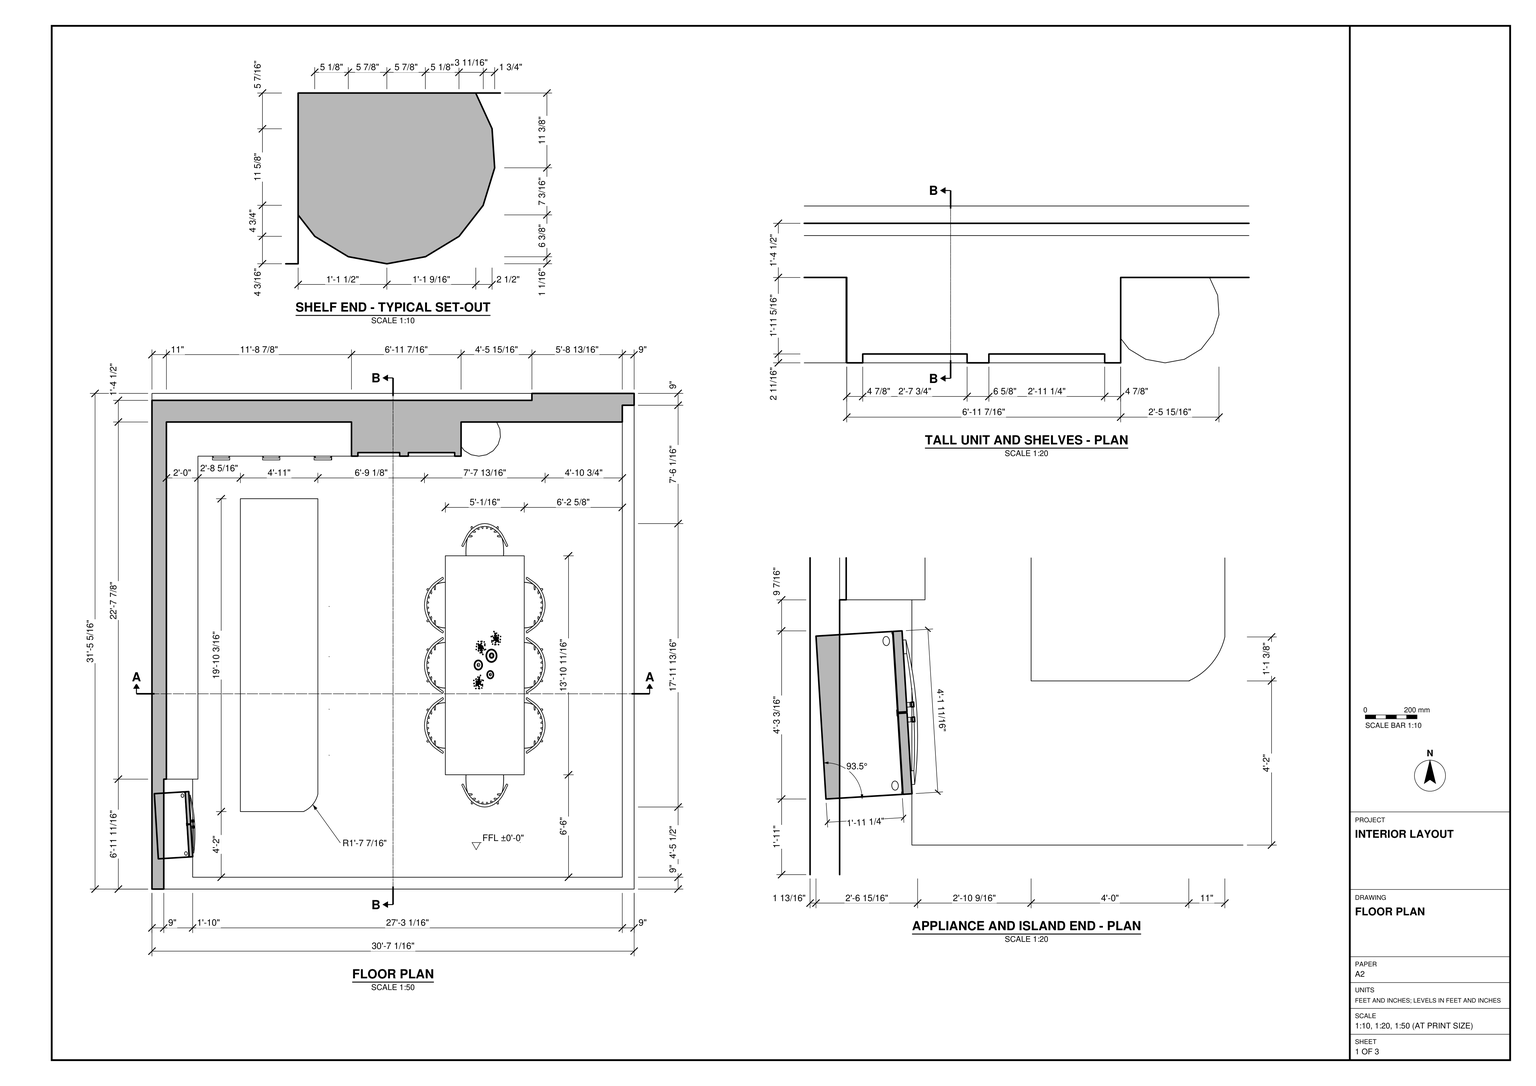
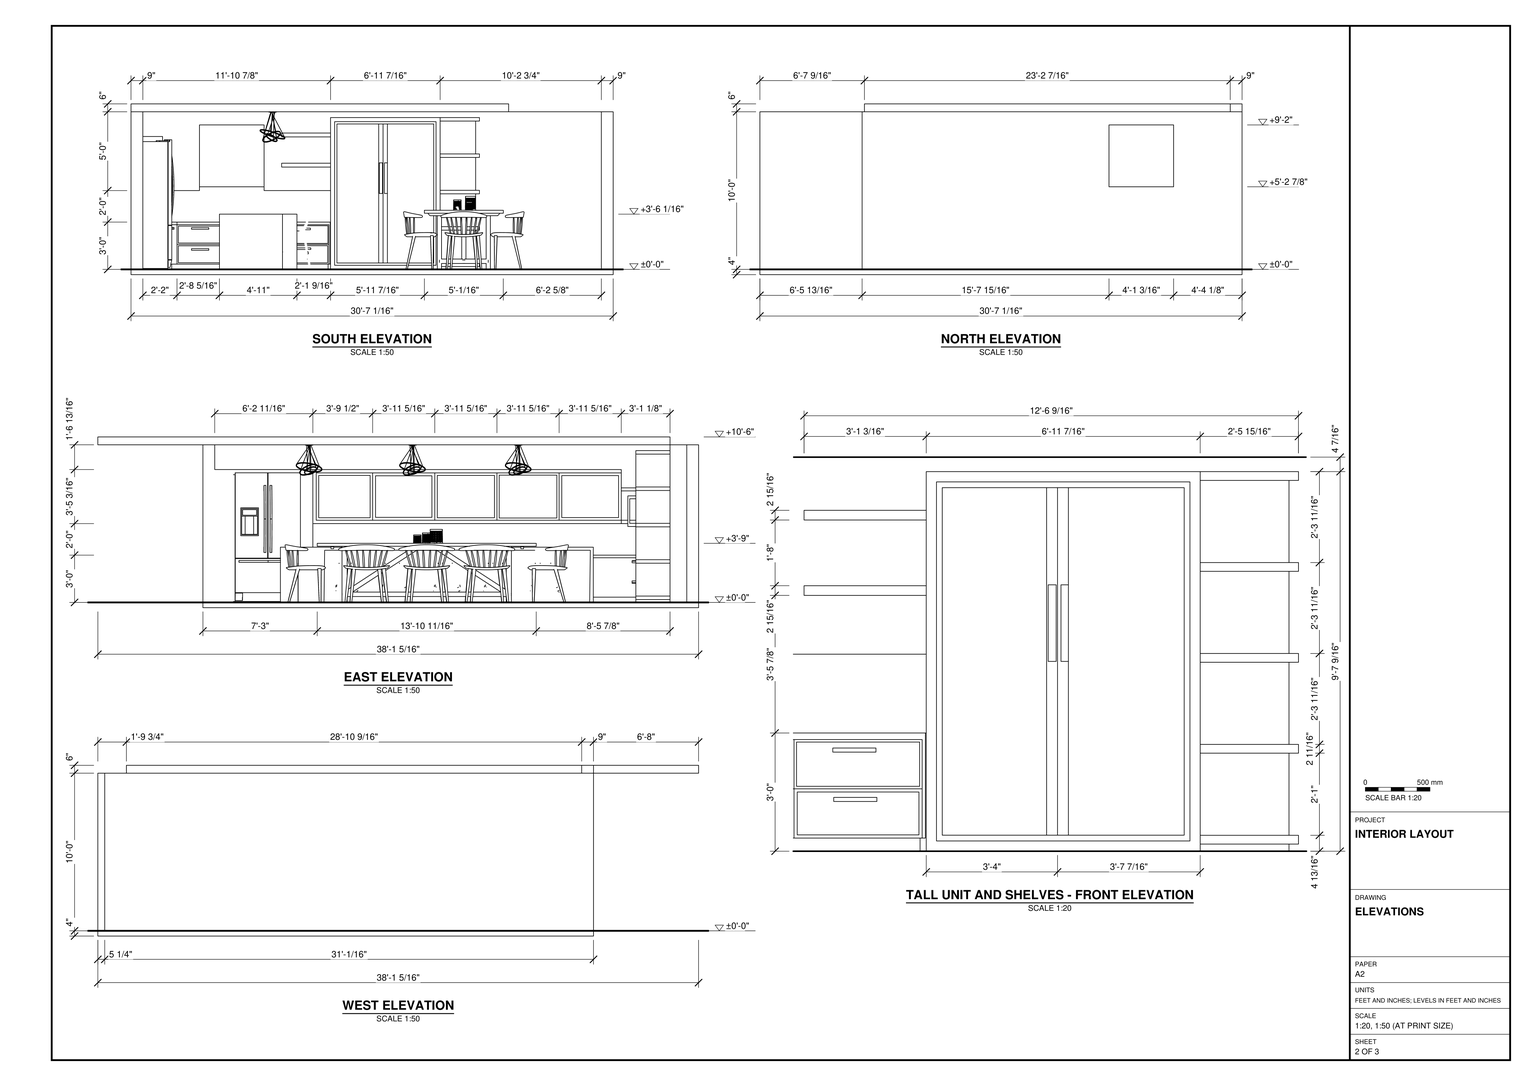
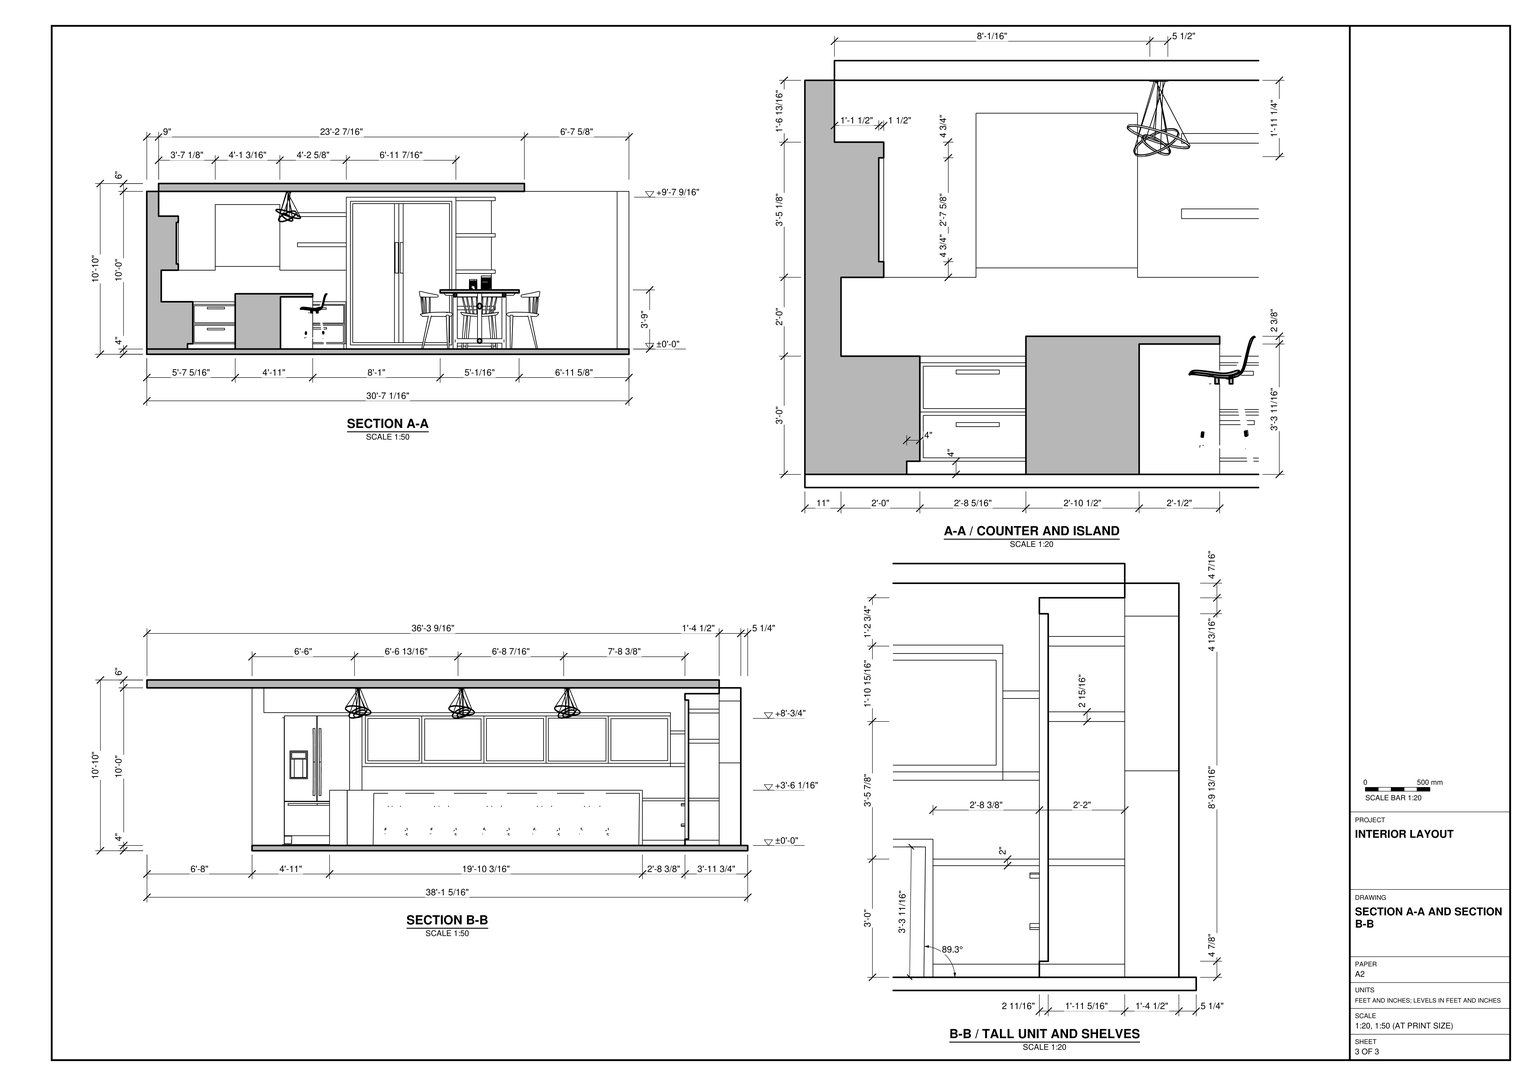
Build the kitchen and dining interior in SketchUp from task_files/diagram_01.pdf. Work in feet and inches. Set the finished floor at ±0'-0". The overall model measures 30'-7 1/16" along X, 38'-1 5/16" along Y and 10'-10" along Z. Use the plan for the room footprint and wall thicknesses, and the sections for the floor slab, wall heights and projecting overhead slab. Retain the open sides shown in the elevations and the rectangular opening in the north wall.

Lay out the wall counter, drawers, upper cabinets and refrigerator along the west side. On the north side, model the tall double-door unit with its handles, low drawers and flanking shelves. Use the enlarged shelf-end plan to shape the exposed shelf ends. Set the island parallel to the west counter, leaving the aisle shown in section A-A. Reproduce the island's rounded corner and projecting top, with stools on the dining side and pendant lights above. Place the dining table parallel to the island, with chairs along both sides and at the ends.

Decor and loose items, including lights, appliances and tabletop objects, may be any suitable library components. Keep shell elements and each furniture or joinery piece in separate groups or components, and use components for repeated parts. Save one SketchUp model as output_files/kitchen_and_dining_room_with_an_island.skp.

# SketchUp Ruby script. Lengths in inches.
U = 1.inch
M = Sketchup.active_model
def pt(a) = Geom::Point3d.new(a.map { |v| v * U })
def face(e, loops, mat)
  f = e.add_face(loops[0].map { |a| pt(a) })
  loops[1..].each { |l| e.add_face(l.map { |a| pt(a) }).erase! }
  f.material = f.back_material = mat if mat
  f
end
# faces: each face lists its corners as indices into pts; further lists are holes
def faces(e, pts, list, mat = nil) = list.each { |f| face(e, (f[0].is_a?(Array) ? f : [f]).map { |l| l.map { |i| pts[i] } }, mat) }
# xy, xz, yz: faces in a plane at the given z, y or x. An outline is a flat list of corners, or four numbers for a rectangle; further outlines are holes
def ring(l) = l.size == 4 ? [[l[0], l[1]], [l[2], l[1]], [l[2], l[3]], [l[0], l[3]]] : l.each_slice(2).to_a
def flat(e, list, mat, &to3) = list.each { |f| face(e, (f[0].is_a?(Array) ? f : [f]).map { |l| ring(l).map { |u, v| to3.(u, v) } }, mat) }
def xy(e, z, list, mat = nil) = flat(e, list, mat) { |x, y| [x, y, z] }
def xz(e, y, list, mat = nil) = flat(e, list, mat) { |x, z| [x, y, z] }
def yz(e, x, list, mat = nil) = flat(e, list, mat) { |y, z| [x, y, z] }
def lines(e, pts, list) = list.each { |a, b| e.add_line(pt(pts[a]), pt(pts[b])) }
# prism: a flat outline (further loops are holes) pulled along v
def prism(e, loops, v, mat = nil)
  f = face(e, loops, mat); d = Geom::Vector3d.new(v.map { |x| x * U })
  f.pushpull(f.normal.samedirection?(d) ? d.length : -d.length)
end
def box(e, o, s, mat = nil) = prism(e, [[o, [o[0] + s[0], o[1], o[2]], [o[0] + s[0], o[1] + s[1], o[2]], [o[0], o[1] + s[1], o[2]]]], [0, 0, s[2]], mat)
def at(x, y, z, deg = 0) = Geom::Transformation.translation(pt([x, y, z])) * Geom::Transformation.rotation(ORIGIN, Z_AXIS, deg.degrees)
def axes(o, x, y, z) = Geom::Transformation.new([*x, 0, *y, 0, *z, 0, *pt(o).to_a, 1])
def part(name) = M.definitions.add(name)
# library, detail: a bought-in or finely detailed component or shape, given as its bounding box
def library(name, o, s) = part(name).tap { |d| box(d.entities, o, s) }
def detail(e, o, s) = box(e.add_group.entities, o, s)
def put(e, d, t, mat = nil) = e.add_instance(d, t).tap { |i| i.material = mat if mat }
def group(e, t, mat = nil) = e.add_group.tap { |g| g.transformation = t; g.material = mat if mat }.entities
root = M.entities
M.materials.add("Generic\#1").color = [245, 202, 215]
M.materials.add("Generic\#2").color = [31, 50, 76]
M.materials.add("Generic\#5").color = [5, 14, 47]
M.materials.add("Generic\#7").color = [251, 187, 251]
M.materials.add("Glass_Basic_01").color = [161, 173, 186]
M.materials["Glass_Basic_01"].alpha = 0.25
M.materials.add("Glass_Safety_01").color = [204, 235, 244]
M.materials["Glass_Safety_01"].alpha = 0.25
M.materials.add("M07_Charcoal_Gleam").color = [58, 58, 58]
M.materials.add("M08_Obsidian_Black").color = [30, 30, 30]
M.materials.add("Plywood_01_1K").color = [125, 96, 64]
M.materials.add("Plywood_08_1K").color = [202, 166, 113]
M.materials.add("[0046_Gold]").color = [155, 138, 35]
M.materials.add("[Color M08]").color = [30, 30, 30]
c1 = part("Groupe\#60")
prism(c1.entities,[[[0.92,0.875,0],[0.92,0.875,0.77],[0.92,0.21,0.77],[0.92,0.21,6.79],[0.92,0.875,6.79],[0.92,0.875,7.5],[0.92,0,7.5],[0.92,0,0]]],[-0.92,0,0])
c2 = part("Groupe\#232")
prism(c2.entities,[[[0.26,0.875,0],[0.26,0.875,0.77],[0.26,0.21,0.77],[0.26,0.21,6.79],[0.26,0.875,6.79],[0.26,0.875,7.5],[0.26,0,7.5],[0.26,0,0]]],[-0.85,0,0])
c3 = part("poignée or")
put(c3.entities,c1,axes([0,0,0],[0.99724,0,0],[0,1,0],[0,0,1]),"[Color M08]")
put(c3.entities,c2,axes([2.0625,0,0],[0.99724,0,0],[0,1,0],[0,0,1]),"[Color M08]")
c4 = part("Door handles gold")
prism(c4.entities,[[[0.79,1.97,-1.97],[0.79,0.79,-1.97],[14.96,0.79,-1.97],[14.96,1.97,-1.97],[15.75,1.97,-1.97],[15.75,0,-1.97],[0,0,-1.97],[0,1.97,-1.97]]],[0,0,1.97],"[0046_Gold]")
c5 = library("Bar stool1",[106.6,-42.125,0],[19.2,20.36,33.82])
c6 = library("Mika Dining Table\#1",[0,0,0],[64.21,124.27,37.09])
c7 = library("Lustre Camila",[-20.78,-21.03,-37.89],[41.37,42.29,37.89])
c8 = library("French door refrigerator",[0,0,0],[35.5,29.25,69.5])
xy(root,4,[[9,80,367.05,80,367.05,448.34,358.05,448.34,358.05,89,31,89,31,163.6875,9,163.6875],[115.3,138.99,116.64,139.66,117.93,140.42,119.15,141.28,120.31,142.24,121.38,143.28,122.375,144.4,123.28,145.59,124.09,146.85,124.8,148.17,125.41,149.53,125.91,150.94,126.3,152.39,126.3,152.48,115.3,152.48],[67.31,152.48,67.31,377.19,126.3,377.19,126.3,374.41,101.78,374.41,101.78,172.17,126.3,172.17,126.3,152.48],[9,163.6875,31,448.34],[151.89,409.58,151.89,435.58,150.01,435.58,150.01,413.58,31,413.58,31,448.34,358.05,448.34,358.05,435.58,235.3125,435.58,235.3125,409.58],
  [0,452.07,289.23,457.34]])
xy(root,6.17,[[248.83,409.58,242.96,410.66,237.85,413.76,235.3125,417.02,235.3125,435.58,262.35,435.58,264.84,430.15,265.24,424.1875,263.49,418.48,259.82,413.76,254.71,410.66]])
xy(root,8,[[31,163.6875,35,413.58],[35,409.58,151.63,413.58],[150.01,413.58,151.63,435.58]])
xy(root,8.84,[[248.83,409.58,254.71,410.66,259.82,413.76,263.49,418.48,265.24,424.1875,264.84,430.15,262.35,435.58,235.3125,435.58,235.3125,417.02,237.85,413.76,242.96,410.66]],"Plywood_08_1K")
xy(root,8.875,[[156.77,409.58,188.55,412.27],[195.18,409.58,230.4375,412.27]])
xy(root,8.91,[[74.23,409.58,110.72,410.45]])
xy(root,8.97,[[112.61,409.58,149.67,410.45]])
xy(root,9.04,[[36.04,409.58,72.28,410.45]])
xy(root,21.96,[[36.04,409.58,72.28,410.45]])
xy(root,22.03,[[112.61,409.58,149.67,410.45]])
xy(root,22.09,[[74.23,409.58,110.72,410.45]])
xy(root,23.66,[[74.2,409.58,110.97,410.45]])
xy(root,23.76,[[112.4,409.58,149.88,410.45]])
xy(root,24.05,[[36.05,409.58,72.27,410.45]])
xy(root,33.85,[[248.83,409.58,242.96,410.66,237.85,413.76,235.3125,417.02,235.3125,435.58,262.35,435.58,264.84,430.15,265.24,424.1875,263.49,418.48,259.82,413.76,254.71,410.66]],"Plywood_08_1K")
xy(root,36.53,[[248.83,409.58,254.71,410.66,259.82,413.76,263.49,418.48,265.24,424.1875,264.84,430.15,262.35,435.58,235.3125,435.58,235.3125,417.02,237.85,413.76,242.96,410.66]],"Plywood_08_1K")
xy(root,36.95,[[36.05,409.58,72.27,410.45]])
xy(root,37.24,[[112.4,409.58,149.88,410.45]])
xy(root,37.34,[[74.2,409.58,110.97,410.45]])
xy(root,40,[[11,163.6875,35,163.6875,35,409.58,151.63,409.58,151.63,435.58,11,435.58]])
xy(root,43.7,[[101.78,172.66,126.3,374.91]])
xy(root,46.05,[[67.31,138.99,115.3,138.99,116.64,139.66,117.93,140.42,119.15,141.28,120.31,142.24,121.38,143.28,122.375,144.4,123.28,145.59,124.09,146.85,124.8,148.17,125.41,149.53,125.91,150.94,126.3,152.39,126.3,377.19,67.31,377.19]])
xy(root,61.54,[[248.83,409.58,242.96,410.66,237.85,413.76,235.3125,417.02,235.3125,435.58,262.35,435.58,264.84,430.15,265.24,424.1875,263.49,418.48,259.82,413.76,254.71,410.66]],"Plywood_08_1K")
xy(root,64,[[11,163.6875,11,401.01,24,398.46,24,163.6875],[24,398.46,11,401.01,11,435.58,24,435.58]])
xy(root,64.21,[[248.83,409.58,254.71,410.66,259.82,413.76,263.49,418.48,265.24,424.1875,264.84,430.15,262.35,435.58,235.3125,435.58,235.3125,417.02,237.85,413.76,242.96,410.66]],"Plywood_08_1K")
xy(root,66.57,[[0.9,398.46,24,435.58]],"Plywood_08_1K")
xy(root,66.88,[[52.11,435.58,101.29,452.07]])
xy(root,68.28,[[22.49,305.54,24,349.4375]])
xy(root,68.46,[[22.49,258.41,24,301.94]])
xy(root,68.48,[[22.49,168.16,24,207.3]])
xy(root,68.6,[[22.49,353.18,24,396.42]])
xy(root,68.77,[[22.49,211.41,24,254.32]])
xy(root,81.9,[[114.6875,409.58,151.89,435.58]])
xy(root,84.85,[[114.6875,409.58,151.89,435.58]],"Plywood_08_1K")
xy(root,88.91,[[0.9,398.46,24,435.58]])
xy(root,89.22,[[248.83,409.58,242.96,410.66,237.85,413.76,235.3125,417.02,235.3125,435.58,262.35,435.58,264.84,430.15,265.24,424.1875,263.49,418.48,259.82,413.76,254.71,410.66]],"Plywood_08_1K")
xy(root,91.22,[[9,398.46,24,435.58]],"Plywood_08_1K")
xy(root,91.9,[[248.83,409.58,254.71,410.66,259.82,413.76,263.49,418.48,265.24,424.1875,264.84,430.15,262.35,435.58,235.3125,435.58,235.3125,417.02,237.85,413.76,242.96,410.66]],"Plywood_08_1K")
xy(root,100.41,[[22.49,211.41,24,254.32]])
xy(root,100.57,[[22.49,353.18,24,396.42]])
xy(root,100.7,[[22.49,168.16,24,207.3]])
xy(root,100.72,[[22.49,258.41,24,301.94]])
xy(root,100.9,[[22.49,305.54,24,349.4375]])
xy(root,104.86,[[114.6875,409.58,151.89,435.58]])
xy(root,105.17,[[9,163.6875,24,398.46]])
xy(root,107.81,[[114.6875,409.58,151.89,435.58]],"Plywood_08_1K")
xy(root,113.99,[[52.11,435.58,101.29,452.07]])
xy(root,114.71,[[156.77,409.58,188.55,412.27],[195.18,409.58,230.4375,412.27]])
xy(root,116.91,[[248.83,409.58,242.96,410.66,237.85,413.76,235.3125,417.02,235.3125,435.58,262.35,435.58,264.84,430.15,265.24,424.1875,263.49,418.48,259.82,413.76,254.71,410.66]],"Plywood_08_1K")
xy(root,119.58,[[151.89,409.58,235.3125,435.58]],"Generic\#2")
xy(root,119.58,[[248.83,409.58,254.71,410.66,259.82,413.76,263.49,418.48,265.24,424.1875,264.84,430.15,262.35,435.58,235.3125,435.58,235.3125,417.02,237.85,413.76,242.96,410.66]],"Plywood_08_1K")
xy(root,124,[[0,0,0,80,9,80,9,435.58,287.46,435.58,287.46,0],[0,80,9,80,9,435.58,150.85,435.58,150.85,452.07,0,452.07],[150.85,435.58,358.05,435.58,358.05,448.34,367.05,448.34,367.05,457.34,289.23,457.34,289.23,452.07,150.85,452.07]])
xy(root,130,[[0,0,287.46,0,287.46,435.58,9,435.58,9,80,0,80]])
xz(root,0,[[0,124,287.46,130]])
xz(root,80,[[0,4,9,124],[0,124,9,130]])
xz(root,138.99,[[67.31,4,115.3,46.05]],"Generic\#7")
xz(root,163.6875,[[9,4,31,8],[9,8,35,38],[9,38,35,40],[9,40,11,64],[9,64,24,105.17]])
xz(root,168.16,[[22.49,68.48,24,100.7]])
xz(root,207.3,[[22.49,68.48,24,100.7]])
xz(root,211.41,[[22.49,68.77,24,100.41]])
xz(root,254.32,[[22.49,68.77,24,100.41]])
xz(root,258.41,[[22.49,68.46,24,100.72]])
xz(root,301.94,[[22.49,68.46,24,100.72]])
xz(root,305.54,[[22.49,68.28,24,100.9]])
xz(root,349.4375,[[22.49,68.28,24,100.9]])
xz(root,353.18,[[22.49,68.6,24,100.57]])
xz(root,377.19,[[67.31,4,126.3,46.05]])
xz(root,396.42,[[22.49,68.6,24,100.57]])
xz(root,398.46,[[0.9,66.57,24,88.91],[9,91.22,24,105.17]])
xz(root,409.58,[[[151.89,4,235.3125,119.58],[155.01,7.12,232.2,116.47]],[[155.01,7.12,232.2,116.47],[156.77,8.875,230.4375,114.71]],[150.64,8,151.63,8,151.63,40,35,40,35,38,150.64,38],[[35,8,73.32,23],[36.04,9.04,72.28,21.96]],[[73.32,8,111.64,23],[74.23,8.91,110.72,22.09]],
  [[111.64,8,150.64,23],[112.61,8.97,149.67,22.03]],[188.55,8.875,191.86,114.71],[191.86,8.875,195.18,114.71],[[35,23,73.32,38],[36.05,24.05,72.27,36.95]],[[73.32,23,111.64,38],[74.2,23.66,110.97,37.34]],
  [[111.64,23,150.64,38],[112.4,23.76,149.88,37.24]]],"Generic\#5")
xz(root,409.58,[[114.6875,81.9,151.89,84.85],[114.6875,104.86,151.89,107.81]],"Plywood_08_1K")
xz(root,410.45,[[74.23,8.91,110.72,22.09],[112.61,8.97,149.67,22.03],[36.04,9.04,72.28,21.96],[74.2,23.66,110.97,37.34],[112.4,23.76,149.88,37.24],
  [36.05,24.05,72.27,36.95]],"Generic\#5")
xz(root,412.27,[[156.77,8.875,188.55,114.71],[195.18,8.875,230.4375,114.71]],"Generic\#5")
xz(root,413.58,[[31,4,150.01,8]],"Generic\#5")
xz(root,435.58,[[262.35,4,358.05,4,358.05,124,9,124,9,91.22,24,91.22,24,88.91,0.9,88.91,0.9,66.57,24,66.57,24,64,52.11,64,52.11,113.99,101.29,113.99,101.29,64,151.89,64,151.89,81.9,114.6875,81.9,114.6875,84.85,151.89,84.85,151.89,104.86,114.6875,104.86,114.6875,107.81,151.89,107.81,151.89,119.58,235.3125,119.58,235.3125,116.91,262.35,116.91],[150.01,4,151.89,4,151.89,40,151.63,40,151.63,8,150.01,8],[9,124,287.46,130]])
xz(root,435.58,[[11,40,151.89,40,151.89,64,101.29,64,101.29,66.88,52.11,66.88,52.11,64,11,64]],"Generic\#1")
xz(root,435.58,[[235.3125,4,262.35,6.17],[235.3125,6.17,262.35,33.85],[235.3125,33.85,262.35,61.54],[235.3125,61.54,262.35,89.22],[235.3125,89.22,262.35,116.91]],"Plywood_08_1K")
xz(root,448.34,[[358.05,4,367.05,124]])
xz(root,452.07,[[[0,4,289.23,124],[52.11,66.88,101.29,113.99]]])
xz(root,452.07,[[52.11,66.88,101.29,113.99]],"Glass_Basic_01")
xz(root,457.34,[[289.23,4,367.05,124]])
yz(root,0,[[80,4,452.07,124],[0,124,80,130]])
yz(root,0.9,[[398.46,66.57,435.58,88.91]])
yz(root,9,[[80,4,163.6875,4,163.6875,105.17,89,105.17,89,124,80,124],[398.46,91.22,435.58,91.22,435.58,124,89,124,89,105.17,398.46,105.17],[80,124,89,130],[89,124,435.58,130]])
yz(root,11,[[163.6875,40,435.58,64]],"Generic\#1")
yz(root,22.49,[[305.54,68.28,349.4375,100.9],[258.41,68.46,301.94,100.72],[168.16,68.48,207.3,100.7],[353.18,68.6,396.42,100.57],[211.41,68.77,254.32,100.41]],"Glass_Safety_01")
yz(root,24,[[[166.25,66.57,209.21,102.61],[168.16,68.48,207.3,100.7]],[[209.21,66.57,256.52,102.61],[211.41,68.77,254.32,100.41]],[[256.52,66.57,303.83,102.61],[258.41,68.46,301.94,100.72]],[[303.83,66.57,351.15,102.61],[305.54,68.28,349.4375,100.9]],[[351.15,66.57,398.46,102.61],[353.18,68.6,396.42,100.57]]],"M07_Charcoal_Gleam")
yz(root,24,[[163.6875,64,398.46,64,398.46,66.57,166.25,66.57,166.25,102.61,398.46,102.61,398.46,105.17,163.6875,105.17]],"M08_Obsidian_Black")
yz(root,24,[[398.46,64,435.58,66.57],[398.46,88.91,435.58,91.22]],"Plywood_08_1K")
yz(root,31,[[163.6875,4,413.58,8]])
yz(root,35,[[163.6875,8,409.58,38],[163.6875,38,409.58,40]])
yz(root,36.04,[[409.58,9.04,410.45,21.96]],"Generic\#5")
yz(root,36.05,[[409.58,24.05,410.45,36.95]],"Generic\#5")
yz(root,52.11,[[435.58,66.88,452.07,113.99]])
yz(root,67.31,[[138.99,4,377.19,46.05]])
yz(root,72.27,[[409.58,24.05,410.45,36.95]])
yz(root,72.28,[[409.58,9.04,410.45,21.96]])
yz(root,74.2,[[409.58,23.66,410.45,37.34]])
yz(root,74.23,[[409.58,8.91,410.45,22.09]])
yz(root,101.29,[[435.58,66.88,452.07,113.99]])
yz(root,101.78,[[172.17,4,374.41,4,374.91,43.7,172.66,43.7]],"Plywood_08_1K")
yz(root,110.72,[[409.58,8.91,410.45,22.09]])
yz(root,110.97,[[409.58,23.66,410.45,37.34]])
yz(root,112.4,[[409.58,23.76,410.45,37.24]])
yz(root,112.61,[[409.58,8.97,410.45,22.03]])
yz(root,114.6875,[[409.58,81.9,435.58,84.85],[409.58,104.86,435.58,107.81]],"Plywood_08_1K")
yz(root,126.3,[[152.39,4,152.48,46.05]])
yz(root,126.3,[[152.48,4,172.17,4,172.66,43.7,374.91,43.7,374.41,4,377.19,4,377.19,46.05,152.48,46.05]],"Generic\#7")
yz(root,149.67,[[409.58,8.97,410.45,22.03]])
yz(root,149.88,[[409.58,23.76,410.45,37.24]])
yz(root,150.01,[[413.58,4,435.58,8]],"Generic\#5")
yz(root,151.63,[[409.58,38,435.58,40]])
yz(root,151.63,[[409.58,8,435.58,38]],"Generic\#5")
yz(root,151.89,[[409.58,4,435.58,81.9],[409.58,84.85,435.58,104.86],[409.58,107.81,435.58,119.58]])
yz(root,156.77,[[409.58,8.875,412.27,114.71]])
yz(root,188.55,[[409.58,8.875,412.27,114.71]])
yz(root,195.18,[[409.58,8.875,412.27,114.71]])
yz(root,230.4375,[[409.58,8.875,412.27,114.71]])
yz(root,235.3125,[[417.02,6.17,435.58,8.84],[417.02,33.85,435.58,36.53],[417.02,61.54,435.58,64.21],[417.02,89.22,435.58,91.9],[417.02,116.91,435.58,119.58]])
yz(root,235.3125,[[409.58,4,435.58,4,435.58,6.17,417.02,6.17,417.02,8.84,435.58,8.84,435.58,33.85,417.02,33.85,417.02,36.53,435.58,36.53,435.58,61.54,417.02,61.54,417.02,64.21,435.58,64.21,435.58,89.22,417.02,89.22,417.02,91.9,435.58,91.9,435.58,116.91,417.02,116.91,417.02,119.58,409.58,119.58]],"Plywood_08_1K")
yz(root,287.46,[[0,124,435.58,130]])
yz(root,289.23,[[452.07,4,457.34,124]])
yz(root,358.05,[[435.58,4,448.34,124]])
yz(root,367.05,[[448.34,4,457.34,124]])
p = [[115.3,138.99,46.05],[116.64,139.66,46.05],[116.64,139.66,4],[115.3,138.99,4],[115.3,138.99,17.28],[117.93,140.42,46.05],
  [117.93,140.42,4],[119.15,141.28,46.05],[119.15,141.28,4],[120.31,142.24,46.05],[120.31,142.24,4],[121.38,143.28,46.05],
  [121.38,143.28,4],[122.375,144.4,46.05],[122.375,144.4,4],[123.28,145.59,46.05],[123.28,145.59,4],[124.09,146.85,46.05],
  [124.09,146.85,4],[124.8,148.17,46.05],[124.8,148.17,4],[125.41,149.53,46.05],[125.41,149.53,4],[125.91,150.94,46.05],
  [125.91,150.94,4],[126.3,152.39,46.05],[126.3,152.39,4],[126.3,172.66,43.7],[126.3,172.17,4],[101.78,172.17,4],
  [101.78,172.66,43.7],[126.3,374.41,4],[126.3,374.91,43.7],[101.78,374.91,43.7],[101.78,374.41,4],[248.83,409.58,8.84],
  [242.96,410.66,8.84],[242.96,410.66,6.17],[248.83,409.58,6.17],[254.71,410.66,8.84],[254.71,410.66,6.17],[237.85,413.76,8.84],
  [237.85,413.76,6.17],[259.82,413.76,8.84],[259.82,413.76,6.17],[235.3125,417.02,8.84],[235.3125,417.02,6.17],[263.49,418.48,8.84],
  [263.49,418.48,6.17],[265.24,424.1875,8.84],[265.24,424.1875,6.17],[264.84,430.15,8.84],[264.84,430.15,6.17],[262.35,435.58,8.84],
  [262.35,435.58,6.17],[248.83,409.58,36.53],[242.96,410.66,36.53],[242.96,410.66,33.85],[248.83,409.58,33.85],[254.71,410.66,36.53],
  [254.71,410.66,33.85],[237.85,413.76,36.53],[237.85,413.76,33.85],[259.82,413.76,36.53],[259.82,413.76,33.85],[235.3125,417.02,36.53],
  [235.3125,417.02,33.85],[263.49,418.48,36.53],[263.49,418.48,33.85],[265.24,424.1875,36.53],[265.24,424.1875,33.85],[264.84,430.15,36.53],
  [264.84,430.15,33.85],[262.35,435.58,36.53],[262.35,435.58,33.85],[248.83,409.58,64.21],[242.96,410.66,64.21],[242.96,410.66,61.54],
  [248.83,409.58,61.54],[254.71,410.66,64.21],[254.71,410.66,61.54],[237.85,413.76,64.21],[237.85,413.76,61.54],[259.82,413.76,64.21],
  [259.82,413.76,61.54],[235.3125,417.02,64.21],[235.3125,417.02,61.54],[263.49,418.48,64.21],[263.49,418.48,61.54],[265.24,424.1875,64.21],
  [265.24,424.1875,61.54],[264.84,430.15,64.21],[264.84,430.15,61.54],[262.35,435.58,64.21],[262.35,435.58,61.54],[248.83,409.58,91.9],
  [242.96,410.66,91.9],[242.96,410.66,89.22],[248.83,409.58,89.22],[254.71,410.66,91.9],[254.71,410.66,89.22],[237.85,413.76,91.9],
  [237.85,413.76,89.22],[259.82,413.76,91.9],[259.82,413.76,89.22],[235.3125,417.02,91.9],[235.3125,417.02,89.22],[263.49,418.48,91.9],
  [263.49,418.48,89.22],[265.24,424.1875,91.9],[265.24,424.1875,89.22],[264.84,430.15,91.9],[264.84,430.15,89.22],[262.35,435.58,91.9],
  [262.35,435.58,89.22],[248.83,409.58,119.58],[242.96,410.66,119.58],[242.96,410.66,116.91],[248.83,409.58,116.91],[254.71,410.66,119.58],
  [254.71,410.66,116.91],[237.85,413.76,119.58],[237.85,413.76,116.91],[259.82,413.76,119.58],[259.82,413.76,116.91],[235.3125,417.02,119.58],
  [235.3125,417.02,116.91],[263.49,418.48,119.58],[263.49,418.48,116.91],[265.24,424.1875,119.58],[265.24,424.1875,116.91],[264.84,430.15,119.58],
  [264.84,430.15,116.91],[262.35,435.58,119.58],[262.35,435.58,116.91],[115.53,138.99,4],[115.53,138.99,17.28],[115.3,152.48,46.05],
  [115.3,152.48,4]]
faces(root,p,[[0,1,2,3,4],[1,5,6,2],[5,7,8,6],[7,9,10,8],[9,11,12,10],[11,13,14,12],[13,15,16,14],[15,17,18,16],
  [17,19,20,18],[19,21,22,20],[21,23,24,22],[23,25,26,24]],"Generic\#7")
faces(root,p,[[27,28,29,30],[31,32,33,34]])
faces(root,p,[[35,36,37,38],[39,35,38,40],[36,41,42,37],[43,39,40,44],[41,45,46,42],[47,43,44,48],[49,47,48,50],[51,49,50,52],
  [53,51,52,54],[55,56,57,58],[59,55,58,60],[56,61,62,57],[63,59,60,64],[61,65,66,62],[67,63,64,68],[69,67,68,70],
  [71,69,70,72],[73,71,72,74],[75,76,77,78],[79,75,78,80],[76,81,82,77],[83,79,80,84],[81,85,86,82],[87,83,84,88],
  [89,87,88,90],[91,89,90,92],[93,91,92,94],[95,96,97,98],[99,95,98,100],[96,101,102,97],[103,99,100,104],[101,105,106,102],
  [107,103,104,108],[109,107,108,110],[111,109,110,112],[113,111,112,114],[115,116,117,118],[119,115,118,120],[116,121,122,117],[123,119,120,124],
  [121,125,126,122],[127,123,124,128],[129,127,128,130],[131,129,130,132],[133,131,132,134]],"Plywood_08_1K")
lines(root,p,[[135,3],[4,136],[137,138]])
put(root,c3,axes([189.02,403.49,61.79],[2.65218,0,0],[0,6.9646,0],[0,0,3.1104]))
put(root,c4,axes([123.4375,406.7,35.42],[0.83429,0,0],[0,1.90957,0],[0,0,0.63101]))
put(root,c4,axes([123.72,406.7,20.39],[0.83429,0,0],[0,1.90957,0],[0,0,0.63101]))
put(root,c4,axes([84.23,406.7,20.39],[0.83429,0,0],[0,1.90957,0],[0,0,0.63101]))
put(root,c4,axes([84.23,406.7,35.79],[0.83429,0,0],[0,1.90957,0],[0,0,0.63101]))
put(root,c4,axes([46.06,406.7,35.79],[0.83429,0,0],[0,1.90957,0],[0,0,0.63101]))
put(root,c4,axes([46.06,406.7,19.78],[0.83429,0,0],[0,1.90957,0],[0,0,0.63101]))
put(root,c5,axes([159.15,388.82,4],[0,-1.4022,0],[1,0,0],[0,0,1.24353]))
put(root,c5,axes([159.15,431.88,4],[0,-1.4268,0],[1,0,0],[0,0,1.24353]))
put(root,c5,axes([159.15,521.02,4],[0,-1.55165,0],[1,0,0],[0,0,1.24353]))
put(root,c5,axes([159.15,470.08,4],[0,-1.4268,0],[1,0,0],[0,0,1.24353]))
put(root,c5,axes([159.15,332.68,4],[0,-1.23,0],[1,0,0],[0,0,1.24353]))
put(root,c6,axes([207.45,142.48,4],[1.43,0,0],[0,1.7365,0],[0,0,1.5]))
put(root,c7,axes([107.77,160.74,124],[0.65,0,0],[0,0.65,0],[0,0,0.65]))
put(root,c7,axes([107.77,239.46,124],[0.65,0,0],[0,0.65,0],[0,0,0.65]))
put(root,c7,axes([107.77,319.96,124],[0.65,0,0],[0,0.65,0],[0,0,0.65]))
put(root,c8,axes([1.8,152.64,4],[0.08533,-1.3974,0],[0.99814,0.06095,0],[0,0,1.42]))
g1 = group(root,at(0,80,0),"Plywood_08_1K")
xy(g1,0,[[0,0,367.05,377.34]])
xy(g1,4,[[0,0,367.05,377.34]],"Plywood_01_1K")
xz(g1,0,[[0,0,367.05,4]])
xz(g1,377.34,[[0,0,367.05,4]])
yz(g1,0,[[0,0,377.34,4]])
yz(g1,367.05,[[0,0,377.34,4]])
